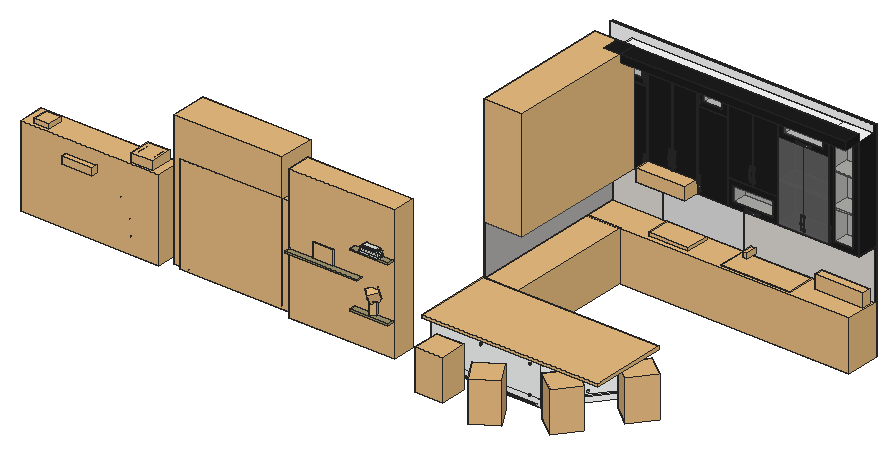
# SketchUp Ruby script. Lengths in inches.
U = 1.inch
M = Sketchup.active_model
def pt(a) = Geom::Point3d.new(a.map { |v| v * U })
def face(e, loops, mat)
  f = e.add_face(loops[0].map { |a| pt(a) })
  loops[1..].each { |l| e.add_face(l.map { |a| pt(a) }).erase! }
  f.material = f.back_material = mat if mat
  f
end
# faces: each face lists its corners as indices into pts; further lists are holes
def faces(e, pts, list, mat = nil) = list.each { |f| face(e, (f[0].is_a?(Array) ? f : [f]).map { |l| l.map { |i| pts[i] } }, mat) }
# xy, xz, yz: faces in a plane at the given z, y or x. An outline is a flat list of corners, or four numbers for a rectangle; further outlines are holes
def ring(l) = l.size == 4 ? [[l[0], l[1]], [l[2], l[1]], [l[2], l[3]], [l[0], l[3]]] : l.each_slice(2).to_a
def flat(e, list, mat, &to3) = list.each { |f| face(e, (f[0].is_a?(Array) ? f : [f]).map { |l| ring(l).map { |u, v| to3.(u, v) } }, mat) }
def xy(e, z, list, mat = nil) = flat(e, list, mat) { |x, y| [x, y, z] }
def xz(e, y, list, mat = nil) = flat(e, list, mat) { |x, z| [x, y, z] }
def yz(e, x, list, mat = nil) = flat(e, list, mat) { |y, z| [x, y, z] }
def lines(e, pts, list) = list.each { |a, b| e.add_line(pt(pts[a]), pt(pts[b])) }
# prism: a flat outline (further loops are holes) pulled along v
def prism(e, loops, v, mat = nil)
  f = face(e, loops, mat); d = Geom::Vector3d.new(v.map { |x| x * U })
  f.pushpull(f.normal.samedirection?(d) ? d.length : -d.length)
end
def box(e, o, s, mat = nil) = prism(e, [[o, [o[0] + s[0], o[1], o[2]], [o[0] + s[0], o[1] + s[1], o[2]], [o[0], o[1] + s[1], o[2]]]], [0, 0, s[2]], mat)
def at(x, y, z, deg = 0) = Geom::Transformation.translation(pt([x, y, z])) * Geom::Transformation.rotation(ORIGIN, Z_AXIS, deg.degrees)
def axes(o, x, y, z) = Geom::Transformation.new([*x, 0, *y, 0, *z, 0, *pt(o).to_a, 1])
def part(name) = M.definitions.add(name)
# library, detail: a bought-in or finely detailed component or shape, given as its bounding box
def library(name, o, s) = part(name).tap { |d| box(d.entities, o, s) }
def detail(e, o, s) = box(e.add_group.entities, o, s)
def put(e, d, t, mat = nil) = e.add_instance(d, t).tap { |i| i.material = mat if mat }
def group(e, t, mat = nil) = e.add_group.tap { |g| g.transformation = t; g.material = mat if mat }.entities
root = M.entities
M.materials.add("Material1 glass").color = [170, 237, 177]
M.materials["Material1 glass"].alpha = 0.04
M.materials.add("Material1 metal").color = [192, 192, 192]
M.materials.add("Material14 kitchen ceramic").color = [29, 29, 29]
M.materials.add("Material17 ceramic").color = [227, 223, 218]
M.materials.add("Material3 mirror").color = [229, 229, 229]
M.materials.add("Material__1").color = [51, 42, 44]
M.materials.add("Material__2").color = [97, 132, 37]
M.materials.add("[ Metal Corrugated Shiny]1").color = [192, 192, 192]
M.materials.add("[Color_000]").color = [255, 255, 255]
M.materials.add("[Color_D05]").color = [255, 242, 204]
M.materials.add("[Translucent Glass Gray]").color = [128, 128, 128]
M.materials["[Translucent Glass Gray]"].alpha = 0.44
M.materials.add("[Wood Lumber ButtJoined]").color = [164, 152, 112]
M.materials.add("[Wood OSB]").color = [240, 195, 122]
M.materials.add("abu metal").color = [255, 255, 255]
M.materials.add("putih ceramic").color = [255, 255, 255]
c1 = library("1-POIGNEE CLC2",[-3.03,-0.375,0],[6.06,0.75,1.42])
c2 = library("Concrete_Pot_w_Mammilleria_Cactus",[-101.61,-9.94,31.01],[5.9,6.21,9.6])
c3 = library("Untitled",[-1.42,-1.51,0],[11.39,11.39,1.78])
c4 = library("Sphere Light",[-10.3,-10.3,-10.3],[20.6,20.6,20.6])
c5 = library("Plants indoor GHD",[-162.85,0,-1.77],[77.96,22.4,70.79])
c6 = part("Wall cabinet door")
box(c6.entities,[-0.79,0,0],[0.79,17.85,60.24],"Material14 kitchen ceramic")
c7 = part("Component\#352")
box(c7.entities,[0,0,0],[0.79,21.46,61.8125],"Material14 kitchen ceramic")
c8 = part("Wall cabinet door \#1")
box(c8.entities,[-0.79,0,0],[0.79,17.76,72.44],"Material14 kitchen ceramic")
c9 = part("Component\#328")
box(c9.entities,[0,0,0],[11.8125,173.23,5.91],"Material14 kitchen ceramic")
c10 = part("Wall cabinet carcass")
xy(c10.entities,11.38,[[0,0,0,188.98,14.76,188.98,14.76,73.29,0.79,73.29,0.79,37.6,14.76,37.6,14.76,15.75,1.97,15.75,1.97,0],[1.97,0,14.76,15.75],[14.76,0,15.75,14.76]],"Material14 kitchen ceramic")
xy(c10.entities,11.8125,[[0,0,0,188.98,14.76,188.98,14.76,73.29,0.79,73.29,0.79,37.6,14.76,37.6,14.76,15.75,1.97,15.75,1.97,0]],"Material14 kitchen ceramic")
xy(c10.entities,12.68,[[0.98,95.93,14.76,130.25],[0.98,168.31,14.76,188.1875]])
xy(c10.entities,13.54,[[0.98,131.23,14.76,166.94]],"Material14 kitchen ceramic")
xy(c10.entities,19.69,[[0.79,37.6,14.76,73.29]],"Material14 kitchen ceramic")
xy(c10.entities,30.63,[[0.98,95.93,14.76,130.25]])
xy(c10.entities,74.02,[[0.98,131.23,14.76,166.94]],"Material14 kitchen ceramic")
xy(c10.entities,74.88,[[0.98,16.73,14.76,36.61],[0.98,74.28,14.76,94.16],[0.98,132.02,14.76,166.54]],"putih ceramic")
xy(c10.entities,91.26,[[0.98,168.31,14.76,188.1875]])
xy(c10.entities,91.26,[[0.98,16.73,14.76,36.61],[0.98,74.28,14.76,94.16],[0.98,132.02,14.76,166.54]],"putih ceramic")
xy(c10.entities,92.52,[[1.97,15.75,14.76,167.52],[1.97,167.52,14.76,188.98]],"putih ceramic")
xy(c10.entities,98.43,[[0,0,1.97,188.98]],"Material14 kitchen ceramic")
xz(c10.entities,0,[[0,11.38,1.97,11.8125],[1.97,11.38,14.76,11.8125],[14.76,11.38,15.75,11.8125]],"Material14 kitchen ceramic")
xz(c10.entities,0,[[0,11.8125,1.97,98.43]],"putih ceramic")
xz(c10.entities,14.76,[[14.76,11.38,15.75,11.8125]],"abu metal")
xz(c10.entities,15.75,[[1.97,11.38,14.76,11.8125]],"Material14 kitchen ceramic")
xz(c10.entities,15.75,[[1.97,11.8125,14.76,92.52]],"putih ceramic")
xz(c10.entities,16.73,[[0.98,74.88,14.76,91.26]],"putih ceramic")
xz(c10.entities,36.61,[[0.98,74.88,14.76,91.26]],"putih ceramic")
xz(c10.entities,37.6,[[0.79,11.38,14.76,11.8125],[0.79,11.8125,14.76,19.69]],"Material14 kitchen ceramic")
xz(c10.entities,73.29,[[0.79,11.38,14.76,11.8125],[0.79,11.8125,14.76,19.69]],"Material14 kitchen ceramic")
xz(c10.entities,74.28,[[0.98,74.88,14.76,91.26]],"putih ceramic")
xz(c10.entities,94.16,[[0.98,74.88,14.76,91.26]],"putih ceramic")
xz(c10.entities,95.93,[[0.98,12.68,14.76,30.63]])
xz(c10.entities,130.25,[[0.98,12.68,14.76,30.63]])
xz(c10.entities,131.23,[[0.98,13.54,14.76,74.02]],"Material14 kitchen ceramic")
xz(c10.entities,132.02,[[0.98,74.88,14.76,91.26]],"putih ceramic")
xz(c10.entities,166.54,[[0.98,74.88,14.76,91.26]],"putih ceramic")
xz(c10.entities,166.94,[[0.98,13.54,14.76,74.02]],"Material14 kitchen ceramic")
xz(c10.entities,168.31,[[0.98,12.68,14.76,91.26]])
xz(c10.entities,188.1875,[[0.98,12.68,14.76,91.26]])
xz(c10.entities,188.98,[[0,11.38,14.76,11.8125],[0,11.8125,0,98.43,1.97,98.43,1.97,92.52,14.76,92.52,14.76,11.8125]],"Material14 kitchen ceramic")
yz(c10.entities,0,[[0,11.38,188.98,11.8125]],"Material14 kitchen ceramic")
yz(c10.entities,0,[[0,11.8125,188.98,98.43]],"putih ceramic")
yz(c10.entities,0.79,[[37.6,11.38,73.29,11.8125],[37.6,11.8125,73.29,19.69]],"Material14 kitchen ceramic")
yz(c10.entities,0.98,[[95.93,12.68,130.25,30.63],[168.31,12.68,188.1875,91.26]])
yz(c10.entities,0.98,[[131.23,13.54,166.94,74.02]],"Material14 kitchen ceramic")
yz(c10.entities,0.98,[[16.73,74.88,36.61,91.26],[74.28,74.88,94.16,91.26],[132.02,74.88,166.54,91.26]],"putih ceramic")
yz(c10.entities,1.97,[[0,11.38,15.75,11.8125]],"Material14 kitchen ceramic")
yz(c10.entities,1.97,[[0,11.8125,15.75,11.8125,15.75,92.52,188.98,92.52,188.98,98.43,0,98.43]],"putih ceramic")
yz(c10.entities,14.76,[[[95.14,11.8125,131.04,31.5],[95.93,12.68,130.25,30.63]],[[167.52,11.8125,188.98,92.125],[168.31,12.68,188.1875,91.26]]])
yz(c10.entities,14.76,[[166.94,11.38,167.52,11.8125],[131.23,11.8125,166.94,13.54]],"Material14 kitchen ceramic")
yz(c10.entities,14.76,[[14.76,11.38,15.75,11.8125],[15.75,11.38,37.6,11.8125],[73.29,11.38,95.14,11.8125],[95.14,11.38,131.04,11.8125],[131.04,11.38,131.23,11.8125],
  [131.23,11.38,166.94,11.8125],[167.52,11.38,188.98,11.8125]],"abu metal")
yz(c10.entities,14.76,[[[15.75,11.8125,37.6,11.8125,37.6,19.69,73.29,19.69,73.29,11.8125,95.14,11.8125,95.14,31.5,131.04,31.5,131.04,11.8125,131.23,11.8125,131.23,92.125,167.32,92.125,167.32,74.02,166.94,74.02,166.94,11.8125,167.52,11.8125,167.52,92.52,15.75,92.52],[15.94,74.02,37.4,92.125],[73.49,74.02,94.95,92.125]],[[15.94,74.02,37.4,92.125],[16.73,74.88,36.61,91.26]],[[73.49,74.02,94.95,92.125],[74.28,74.88,94.16,91.26]],[[131.23,74.02,167.32,92.125],[132.02,74.88,166.54,91.26]],[167.52,92.125,188.98,92.52]],"putih ceramic")
yz(c10.entities,15.75,[[0,11.38,14.76,11.8125]],"Material14 kitchen ceramic")
c11 = part("Cabinet panel")
box(c11.entities,[-0.79,0,0],[0.4,17.76,62],"[Translucent Glass Gray]")
c12 = library("Bosch-Ventilation-DUH30252UC",[0,-0.03,0],[30,20.53,6.0625])
c13 = part("Framed cabinet door")
xy(c13.entities,5.91,[[-0.79,0,0,21.46]],"Material14 kitchen ceramic")
xy(c13.entities,9.84,[[-0.79,3.9375,-0.39,17.52],[-0.39,3.9375,0,17.52]],"Material14 kitchen ceramic")
xy(c13.entities,82.28,[[-0.79,3.9375,-0.39,17.52],[-0.39,3.9375,0,17.52]],"Material14 kitchen ceramic")
xy(c13.entities,86.22,[[-0.79,0,0,21.46]],"Material14 kitchen ceramic")
xz(c13.entities,0,[[-0.79,5.91,0,86.22]],"Material14 kitchen ceramic")
xz(c13.entities,3.9375,[[-0.79,9.84,-0.39,82.28],[-0.39,9.84,0,82.28]],"Material14 kitchen ceramic")
xz(c13.entities,17.52,[[-0.79,9.84,-0.39,82.28],[-0.39,9.84,0,82.28]],"Material14 kitchen ceramic")
xz(c13.entities,21.46,[[-0.79,5.91,0,86.22]],"Material14 kitchen ceramic")
yz(c13.entities,-0.79,[[[0,5.91,21.46,86.22],[3.9375,9.84,17.52,82.28]]],"Material14 kitchen ceramic")
yz(c13.entities,-0.39,[[3.9375,9.84,17.52,82.28]],"[Translucent Glass Gray]")
yz(c13.entities,0,[[[0,5.91,21.46,86.22],[3.9375,9.84,17.52,82.28]]],"Material14 kitchen ceramic")
c14 = part("Framed cabinet front")
xy(c14.entities,0,[[0,0,0.79,21.46]],"Material14 kitchen ceramic")
xy(c14.entities,3.58,[[0,3.9375,0.39,17.52],[0.39,3.9375,0.79,17.52]],"Material14 kitchen ceramic")
xy(c14.entities,12.88,[[0,3.9375,0.39,17.52],[0.39,3.9375,0.79,17.52]],"Material14 kitchen ceramic")
xy(c14.entities,16.46,[[0,0,0.79,21.46]],"Material14 kitchen ceramic")
xz(c14.entities,0,[[0,0,0.79,16.46]],"Material14 kitchen ceramic")
xz(c14.entities,3.9375,[[0,3.58,0.39,12.88],[0.39,3.58,0.79,12.88]],"Material14 kitchen ceramic")
xz(c14.entities,17.52,[[0,3.58,0.39,12.88],[0.39,3.58,0.79,12.88]],"Material14 kitchen ceramic")
xz(c14.entities,21.46,[[0,0,0.79,16.46]],"Material14 kitchen ceramic")
yz(c14.entities,0,[[[0,0,21.46,16.46],[3.9375,3.58,17.52,12.88]]],"Material14 kitchen ceramic")
yz(c14.entities,0.39,[[3.9375,3.58,17.52,12.88]],"[Translucent Glass Gray]")
yz(c14.entities,0.79,[[[0,0,21.46,16.46],[3.9375,3.58,17.52,12.88]]],"Material14 kitchen ceramic")
c15 = part("Framed cabinet front \#1")
xy(c15.entities,0,[[0,0,0.79,21.46]],"Material14 kitchen ceramic")
xy(c15.entities,3.58,[[0,3.9375,0.39,17.52],[0.39,3.9375,0.79,17.52]],"Material14 kitchen ceramic")
xy(c15.entities,12.88,[[0,3.9375,0.39,17.52],[0.39,3.9375,0.79,17.52]],"Material14 kitchen ceramic")
xy(c15.entities,16.46,[[0,0,0.79,21.46]],"Material14 kitchen ceramic")
xz(c15.entities,0,[[0,0,0.79,16.46]],"Material14 kitchen ceramic")
xz(c15.entities,3.9375,[[0,3.58,0.39,12.88],[0.39,3.58,0.79,12.88]],"Material14 kitchen ceramic")
xz(c15.entities,17.52,[[0,3.58,0.39,12.88],[0.39,3.58,0.79,12.88]],"Material14 kitchen ceramic")
xz(c15.entities,21.46,[[0,0,0.79,16.46]],"Material14 kitchen ceramic")
yz(c15.entities,0,[[[0,0,21.46,16.46],[3.9375,3.58,17.52,12.88]]],"Material14 kitchen ceramic")
yz(c15.entities,0.39,[[3.9375,3.58,17.52,12.88]],"[Translucent Glass Gray]")
yz(c15.entities,0.79,[[[0,0,21.46,16.46],[3.9375,3.58,17.52,12.88]]],"Material14 kitchen ceramic")
c16 = part("Framed cabinet front \#2")
xy(c16.entities,0,[[0,0,0.79,35.89]],"Material14 kitchen ceramic")
xy(c16.entities,3.58,[[0,3.9375,0.39,31.96],[0.39,3.9375,0.79,31.96]],"Material14 kitchen ceramic")
xy(c16.entities,14.32,[[0,3.9375,0.39,31.96],[0.39,3.9375,0.79,31.96]],"Material14 kitchen ceramic")
xy(c16.entities,17.9,[[0,0,0.79,35.89]],"Material14 kitchen ceramic")
xz(c16.entities,0,[[0,0,0.79,17.9]],"Material14 kitchen ceramic")
xz(c16.entities,3.9375,[[0,3.58,0.39,14.32],[0.39,3.58,0.79,14.32]],"Material14 kitchen ceramic")
xz(c16.entities,31.96,[[0,3.58,0.39,14.32],[0.39,3.58,0.79,14.32]],"Material14 kitchen ceramic")
xz(c16.entities,35.89,[[0,0,0.79,17.9]],"Material14 kitchen ceramic")
yz(c16.entities,0,[[[0,0,35.89,17.9],[3.9375,3.58,31.96,14.32]]],"Material14 kitchen ceramic")
yz(c16.entities,0.39,[[3.9375,3.58,31.96,14.32]],"[Translucent Glass Gray]")
yz(c16.entities,0.79,[[[0,0,35.89,17.9],[3.9375,3.58,31.96,14.32]]],"Material14 kitchen ceramic")
c17 = part("Framed cabinet front \#3")
xy(c17.entities,0,[[0,0,0.79,36.09]],"Material14 kitchen ceramic")
xy(c17.entities,3.58,[[0,3.9375,0.39,32.15],[0.39,3.9375,0.79,32.15]],"Material14 kitchen ceramic")
xy(c17.entities,12.88,[[0,3.9375,0.39,32.15],[0.39,3.9375,0.79,32.15]],"Material14 kitchen ceramic")
xy(c17.entities,16.46,[[0,0,0.79,36.09]],"Material14 kitchen ceramic")
xz(c17.entities,0,[[0,0,0.79,16.46]],"Material14 kitchen ceramic")
xz(c17.entities,3.9375,[[0,3.58,0.39,12.88],[0.39,3.58,0.79,12.88]],"Material14 kitchen ceramic")
xz(c17.entities,32.15,[[0,3.58,0.39,12.88],[0.39,3.58,0.79,12.88]],"Material14 kitchen ceramic")
xz(c17.entities,36.09,[[0,0,0.79,16.46]],"Material14 kitchen ceramic")
yz(c17.entities,0,[[[0,0,36.09,16.46],[3.9375,3.58,32.15,12.88]]],"Material14 kitchen ceramic")
yz(c17.entities,0.39,[[3.9375,3.58,32.15,12.88]],"[Translucent Glass Gray]")
yz(c17.entities,0.79,[[[0,0,36.09,16.46],[3.9375,3.58,32.15,12.88]]],"Material14 kitchen ceramic")
c18 = part("Group\#24")
xy(c18.entities,0,[[0,0,35.43,15.75],[0,390.79,35.43,406.54]],"[ Metal Corrugated Shiny]1")
xy(c18.entities,7.09,[[0,0,35.43,15.75],[0,390.79,35.43,406.54]],"[ Metal Corrugated Shiny]1")
xz(c18.entities,0,[[0,0,35.43,7.09]],"[ Metal Corrugated Shiny]1")
xz(c18.entities,406.54,[[0,0,35.43,7.09]],"[ Metal Corrugated Shiny]1")
yz(c18.entities,0,[[0,0,0,7.09,15.75,7.09,21.89,7.25,21.89,0.16,15.75,0],[390.79,0,384.65,0.16,384.65,7.25,390.79,7.09,406.54,7.09,406.54,0],[21.89,0.16,21.89,7.25,28.01,7.7,28.01,0.62],[384.65,0.16,378.53,0.62,378.53,7.7,384.65,7.25],[28.01,0.62,28.01,7.7,34.11,8.45,34.11,1.36],
  [378.53,0.62,372.43,1.36,372.43,8.45,378.53,7.7],[34.11,1.36,34.11,8.45,40.16,9.49,40.16,2.4],[372.43,1.36,366.38,2.4,366.38,9.49,372.43,8.45],[40.16,2.4,40.16,9.49,46.15,10.82,46.15,3.73],[366.38,2.4,360.38,3.73,360.38,10.82,366.38,9.49],
  [46.15,3.73,46.15,10.82,52.08,12.43,52.08,5.34],[360.38,3.73,354.46,5.34,354.46,12.43,360.38,10.82],[52.08,5.34,52.08,12.43,57.92,14.32,57.92,7.24],[354.46,5.34,348.62,7.24,348.62,14.32,354.46,12.43],[57.92,7.24,57.92,14.32,63.66,16.5,63.66,9.41],
  [348.62,7.24,342.875,9.41,342.875,16.5,348.62,14.32],[63.66,9.41,63.66,16.5,69.29,18.94,69.29,11.85],[342.875,9.41,337.24,11.85,337.24,18.94,342.875,16.5],[69.29,11.85,69.29,18.94,74.8,21.65,74.8,14.57],[337.24,11.85,331.73,14.57,331.73,21.65,337.24,18.94],
  [74.8,14.57,74.8,21.65,99.35,31.6,99.35,24.52],[331.73,14.57,307.1875,24.52,307.1875,31.6,331.73,21.65],[99.35,24.52,99.35,31.6,124.66,39.42,124.66,32.33],[307.1875,24.52,281.88,32.33,281.88,39.42,307.1875,31.6],[124.66,32.33,124.66,39.42,150.54,45.04,150.54,37.96],
  [281.88,32.33,256,37.96,256,45.04,281.88,39.42],[150.54,37.96,150.54,45.04,176.81,48.43,176.81,41.35],[256,37.96,229.73,41.35,229.73,48.43,256,45.04],[176.81,41.35,176.81,48.43,203.27,49.57,203.27,42.48],[229.73,41.35,203.27,42.48,203.27,49.57,229.73,48.43]],"[ Metal Corrugated Shiny]1")
yz(c18.entities,35.43,[[0,0,15.75,0,21.89,0.16,21.89,7.25,15.75,7.09,0,7.09],[390.79,0,406.54,0,406.54,7.09,390.79,7.09,384.65,7.25,384.65,0.16],[21.89,0.16,28.01,0.62,28.01,7.7,21.89,7.25],[384.65,0.16,384.65,7.25,378.53,7.7,378.53,0.62],[28.01,0.62,34.11,1.36,34.11,8.45,28.01,7.7],
  [378.53,0.62,378.53,7.7,372.43,8.45,372.43,1.36],[34.11,1.36,40.16,2.4,40.16,9.49,34.11,8.45],[372.43,1.36,372.43,8.45,366.38,9.49,366.38,2.4],[40.16,2.4,46.15,3.73,46.15,10.82,40.16,9.49],[366.38,2.4,366.38,9.49,360.38,10.82,360.38,3.73],
  [46.15,3.73,52.08,5.34,52.08,12.43,46.15,10.82],[360.38,3.73,360.38,10.82,354.46,12.43,354.46,5.34],[52.08,5.34,57.92,7.24,57.92,14.32,52.08,12.43],[354.46,5.34,354.46,12.43,348.62,14.32,348.62,7.24],[57.92,7.24,63.66,9.41,63.66,16.5,57.92,14.32],
  [348.62,7.24,348.62,14.32,342.875,16.5,342.875,9.41],[63.66,9.41,69.29,11.85,69.29,18.94,63.66,16.5],[342.875,9.41,342.875,16.5,337.24,18.94,337.24,11.85],[69.29,11.85,74.8,14.57,74.8,21.65,69.29,18.94],[337.24,11.85,337.24,18.94,331.73,21.65,331.73,14.57],
  [74.8,14.57,99.35,24.52,99.35,31.6,74.8,21.65],[331.73,14.57,331.73,21.65,307.1875,31.6,307.1875,24.52],[99.35,24.52,124.66,32.33,124.66,39.42,99.35,31.6],[307.1875,24.52,307.1875,31.6,281.88,39.42,281.88,32.33],[124.66,32.33,150.54,37.96,150.54,45.04,124.66,39.42],
  [281.88,32.33,281.88,39.42,256,45.04,256,37.96],[150.54,37.96,176.81,41.35,176.81,48.43,150.54,45.04],[256,37.96,256,45.04,229.73,48.43,229.73,41.35],[176.81,41.35,203.27,42.48,203.27,49.57,176.81,48.43],[229.73,41.35,229.73,48.43,203.27,49.57,203.27,42.48]],"[ Metal Corrugated Shiny]1")
p = [[35.43,15.75,0],[0,15.75,0],[0,21.89,0.16],[35.43,21.89,0.16],[35.43,384.65,0.16],[0,384.65,0.16],
  [0,390.79,0],[35.43,390.79,0],[0,28.01,0.62],[35.43,28.01,0.62],[35.43,378.53,0.62],[0,378.53,0.62],
  [0,34.11,1.36],[35.43,34.11,1.36],[35.43,372.43,1.36],[0,372.43,1.36],[0,40.16,2.4],[35.43,40.16,2.4],
  [35.43,366.38,2.4],[0,366.38,2.4],[0,46.15,3.73],[35.43,46.15,3.73],[35.43,360.38,3.73],[0,360.38,3.73],
  [0,52.08,5.34],[35.43,52.08,5.34],[35.43,354.46,5.34],[0,354.46,5.34],[0,57.92,7.24],[35.43,57.92,7.24],
  [35.43,348.62,7.24],[0,348.62,7.24],[0,15.75,7.09],[35.43,15.75,7.09],[35.43,21.89,7.25],[0,21.89,7.25],
  [0,384.65,7.25],[35.43,384.65,7.25],[35.43,390.79,7.09],[0,390.79,7.09],[35.43,28.01,7.7],[0,28.01,7.7],
  [0,63.66,9.41],[35.43,63.66,9.41],[35.43,342.875,9.41],[0,342.875,9.41],[0,378.53,7.7],[35.43,378.53,7.7],
  [35.43,34.11,8.45],[0,34.11,8.45],[0,372.43,8.45],[35.43,372.43,8.45],[35.43,40.16,9.49],[0,40.16,9.49],
  [0,366.38,9.49],[35.43,366.38,9.49],[0,69.29,11.85],[35.43,69.29,11.85],[35.43,337.24,11.85],[0,337.24,11.85],
  [35.43,46.15,10.82],[0,46.15,10.82],[0,360.38,10.82],[35.43,360.38,10.82],[35.43,52.08,12.43],[0,52.08,12.43],
  [0,354.46,12.43],[35.43,354.46,12.43],[0,74.8,14.57],[35.43,74.8,14.57],[35.43,331.73,14.57],[0,331.73,14.57],
  [35.43,57.92,14.32],[0,57.92,14.32],[0,348.62,14.32],[35.43,348.62,14.32],[35.43,63.66,16.5],[0,63.66,16.5],
  [0,342.875,16.5],[35.43,342.875,16.5],[0,99.35,24.52],[35.43,99.35,24.52],[35.43,307.1875,24.52],[0,307.1875,24.52],
  [35.43,69.29,18.94],[0,69.29,18.94],[0,337.24,18.94],[35.43,337.24,18.94],[35.43,74.8,21.65],[0,74.8,21.65],
  [0,331.73,21.65],[35.43,331.73,21.65],[35.43,99.35,31.6],[0,99.35,31.6],[0,307.1875,31.6],[35.43,307.1875,31.6],
  [0,124.66,32.33],[35.43,124.66,32.33],[35.43,281.88,32.33],[0,281.88,32.33],[35.43,124.66,39.42],[0,124.66,39.42],
  [0,281.88,39.42],[35.43,281.88,39.42],[0,150.54,37.96],[35.43,150.54,37.96],[35.43,256,37.96],[0,256,37.96],
  [0,176.81,41.35],[35.43,176.81,41.35],[35.43,229.73,41.35],[0,229.73,41.35],[35.43,150.54,45.04],[0,150.54,45.04],
  [0,256,45.04],[35.43,256,45.04],[0,203.27,42.48],[35.43,203.27,42.48],[35.43,176.81,48.43],[0,176.81,48.43],
  [0,229.73,48.43],[35.43,229.73,48.43],[35.43,203.27,49.57],[0,203.27,49.57]]
faces(c18.entities,p,[[0,1,2,3],[4,5,6,7],[3,2,8,9],[10,11,5,4],[9,8,12,13],[14,15,11,10],[13,12,16,17],[18,19,15,14],
  [17,16,20,21],[22,23,19,18],[21,20,24,25],[26,27,23,22],[25,24,28,29],[30,31,27,26],[32,33,34,35],[36,37,38,39],
  [35,34,40,41],[29,28,42,43],[44,45,31,30],[46,47,37,36],[41,40,48,49],[50,51,47,46],[49,48,52,53],[54,55,51,50],
  [43,42,56,57],[58,59,45,44],[53,52,60,61],[62,63,55,54],[61,60,64,65],[66,67,63,62],[57,56,68,69],[70,71,59,58],
  [65,64,72,73],[74,75,67,66],[73,72,76,77],[78,79,75,74],[69,68,80,81],[82,83,71,70],[77,76,84,85],[86,87,79,78],
  [85,84,88,89],[90,91,87,86],[89,88,92,93],[94,95,91,90],[81,80,96,97],[98,99,83,82],[93,92,100,101],[102,103,95,94],
  [97,96,104,105],[106,107,99,98],[105,104,108,109],[110,111,107,106],[101,100,112,113],[114,115,103,102],[109,108,116,117],[117,116,111,110],
  [113,112,118,119],[120,121,115,114],[119,118,122,123],[123,122,121,120]],"[ Metal Corrugated Shiny]1")
c19 = part("Group\#22")
xy(c19.entities,0,[[0,0,35.43,15.75],[0,390.79,35.43,406.54]],"[ Metal Corrugated Shiny]1")
xy(c19.entities,7.09,[[0,0,35.43,15.75],[0,390.79,35.43,406.54]],"[ Metal Corrugated Shiny]1")
xz(c19.entities,0,[[0,0,35.43,7.09]],"[ Metal Corrugated Shiny]1")
xz(c19.entities,406.54,[[0,0,35.43,7.09]],"[ Metal Corrugated Shiny]1")
yz(c19.entities,0,[[0,0,0,7.09,15.75,7.09,21.89,7.25,21.89,0.16,15.75,0],[390.79,0,384.65,0.16,384.65,7.25,390.79,7.09,406.54,7.09,406.54,0],[21.89,0.16,21.89,7.25,28.01,7.7,28.01,0.62],[384.65,0.16,378.53,0.62,378.53,7.7,384.65,7.25],[28.01,0.62,28.01,7.7,34.11,8.45,34.11,1.36],
  [378.53,0.62,372.43,1.36,372.43,8.45,378.53,7.7],[34.11,1.36,34.11,8.45,40.16,9.49,40.16,2.4],[372.43,1.36,366.38,2.4,366.38,9.49,372.43,8.45],[40.16,2.4,40.16,9.49,46.15,10.82,46.15,3.73],[366.38,2.4,360.38,3.73,360.38,10.82,366.38,9.49],
  [46.15,3.73,46.15,10.82,52.08,12.43,52.08,5.34],[360.38,3.73,354.46,5.34,354.46,12.43,360.38,10.82],[52.08,5.34,52.08,12.43,57.92,14.32,57.92,7.24],[354.46,5.34,348.62,7.24,348.62,14.32,354.46,12.43],[57.92,7.24,57.92,14.32,63.66,16.5,63.66,9.41],
  [348.62,7.24,342.875,9.41,342.875,16.5,348.62,14.32],[63.66,9.41,63.66,16.5,69.29,18.94,69.29,11.85],[342.875,9.41,337.24,11.85,337.24,18.94,342.875,16.5],[69.29,11.85,69.29,18.94,74.8,21.65,74.8,14.57],[337.24,11.85,331.73,14.57,331.73,21.65,337.24,18.94],
  [74.8,14.57,74.8,21.65,99.35,31.6,99.35,24.52],[331.73,14.57,307.1875,24.52,307.1875,31.6,331.73,21.65],[99.35,24.52,99.35,31.6,124.66,39.42,124.66,32.33],[307.1875,24.52,281.88,32.33,281.88,39.42,307.1875,31.6],[124.66,32.33,124.66,39.42,150.54,45.04,150.54,37.96],
  [281.88,32.33,256,37.96,256,45.04,281.88,39.42],[150.54,37.96,150.54,45.04,176.81,48.43,176.81,41.35],[256,37.96,229.73,41.35,229.73,48.43,256,45.04],[176.81,41.35,176.81,48.43,203.27,49.57,203.27,42.48],[229.73,41.35,203.27,42.48,203.27,49.57,229.73,48.43]],"[ Metal Corrugated Shiny]1")
yz(c19.entities,35.43,[[0,0,15.75,0,21.89,0.16,21.89,7.25,15.75,7.09,0,7.09],[390.79,0,406.54,0,406.54,7.09,390.79,7.09,384.65,7.25,384.65,0.16],[21.89,0.16,28.01,0.62,28.01,7.7,21.89,7.25],[384.65,0.16,384.65,7.25,378.53,7.7,378.53,0.62],[28.01,0.62,34.11,1.36,34.11,8.45,28.01,7.7],
  [378.53,0.62,378.53,7.7,372.43,8.45,372.43,1.36],[34.11,1.36,40.16,2.4,40.16,9.49,34.11,8.45],[372.43,1.36,372.43,8.45,366.38,9.49,366.38,2.4],[40.16,2.4,46.15,3.73,46.15,10.82,40.16,9.49],[366.38,2.4,366.38,9.49,360.38,10.82,360.38,3.73],
  [46.15,3.73,52.08,5.34,52.08,12.43,46.15,10.82],[360.38,3.73,360.38,10.82,354.46,12.43,354.46,5.34],[52.08,5.34,57.92,7.24,57.92,14.32,52.08,12.43],[354.46,5.34,354.46,12.43,348.62,14.32,348.62,7.24],[57.92,7.24,63.66,9.41,63.66,16.5,57.92,14.32],
  [348.62,7.24,348.62,14.32,342.875,16.5,342.875,9.41],[63.66,9.41,69.29,11.85,69.29,18.94,63.66,16.5],[342.875,9.41,342.875,16.5,337.24,18.94,337.24,11.85],[69.29,11.85,74.8,14.57,74.8,21.65,69.29,18.94],[337.24,11.85,337.24,18.94,331.73,21.65,331.73,14.57],
  [74.8,14.57,99.35,24.52,99.35,31.6,74.8,21.65],[331.73,14.57,331.73,21.65,307.1875,31.6,307.1875,24.52],[99.35,24.52,124.66,32.33,124.66,39.42,99.35,31.6],[307.1875,24.52,307.1875,31.6,281.88,39.42,281.88,32.33],[124.66,32.33,150.54,37.96,150.54,45.04,124.66,39.42],
  [281.88,32.33,281.88,39.42,256,45.04,256,37.96],[150.54,37.96,176.81,41.35,176.81,48.43,150.54,45.04],[256,37.96,256,45.04,229.73,48.43,229.73,41.35],[176.81,41.35,203.27,42.48,203.27,49.57,176.81,48.43],[229.73,41.35,229.73,48.43,203.27,49.57,203.27,42.48]],"[ Metal Corrugated Shiny]1")
p = [[35.43,15.75,0],[0,15.75,0],[0,21.89,0.16],[35.43,21.89,0.16],[35.43,384.65,0.16],[0,384.65,0.16],
  [0,390.79,0],[35.43,390.79,0],[0,28.01,0.62],[35.43,28.01,0.62],[35.43,378.53,0.62],[0,378.53,0.62],
  [0,34.11,1.36],[35.43,34.11,1.36],[35.43,372.43,1.36],[0,372.43,1.36],[0,40.16,2.4],[35.43,40.16,2.4],
  [35.43,366.38,2.4],[0,366.38,2.4],[0,46.15,3.73],[35.43,46.15,3.73],[35.43,360.38,3.73],[0,360.38,3.73],
  [0,52.08,5.34],[35.43,52.08,5.34],[35.43,354.46,5.34],[0,354.46,5.34],[0,57.92,7.24],[35.43,57.92,7.24],
  [35.43,348.62,7.24],[0,348.62,7.24],[0,15.75,7.09],[35.43,15.75,7.09],[35.43,21.89,7.25],[0,21.89,7.25],
  [0,384.65,7.25],[35.43,384.65,7.25],[35.43,390.79,7.09],[0,390.79,7.09],[35.43,28.01,7.7],[0,28.01,7.7],
  [0,63.66,9.41],[35.43,63.66,9.41],[35.43,342.875,9.41],[0,342.875,9.41],[0,378.53,7.7],[35.43,378.53,7.7],
  [35.43,34.11,8.45],[0,34.11,8.45],[0,372.43,8.45],[35.43,372.43,8.45],[35.43,40.16,9.49],[0,40.16,9.49],
  [0,366.38,9.49],[35.43,366.38,9.49],[0,69.29,11.85],[35.43,69.29,11.85],[35.43,337.24,11.85],[0,337.24,11.85],
  [35.43,46.15,10.82],[0,46.15,10.82],[0,360.38,10.82],[35.43,360.38,10.82],[35.43,52.08,12.43],[0,52.08,12.43],
  [0,354.46,12.43],[35.43,354.46,12.43],[0,74.8,14.57],[35.43,74.8,14.57],[35.43,331.73,14.57],[0,331.73,14.57],
  [35.43,57.92,14.32],[0,57.92,14.32],[0,348.62,14.32],[35.43,348.62,14.32],[35.43,63.66,16.5],[0,63.66,16.5],
  [0,342.875,16.5],[35.43,342.875,16.5],[0,99.35,24.52],[35.43,99.35,24.52],[35.43,307.1875,24.52],[0,307.1875,24.52],
  [35.43,69.29,18.94],[0,69.29,18.94],[0,337.24,18.94],[35.43,337.24,18.94],[35.43,74.8,21.65],[0,74.8,21.65],
  [0,331.73,21.65],[35.43,331.73,21.65],[35.43,99.35,31.6],[0,99.35,31.6],[0,307.1875,31.6],[35.43,307.1875,31.6],
  [0,124.66,32.33],[35.43,124.66,32.33],[35.43,281.88,32.33],[0,281.88,32.33],[35.43,124.66,39.42],[0,124.66,39.42],
  [0,281.88,39.42],[35.43,281.88,39.42],[0,150.54,37.96],[35.43,150.54,37.96],[35.43,256,37.96],[0,256,37.96],
  [0,176.81,41.35],[35.43,176.81,41.35],[35.43,229.73,41.35],[0,229.73,41.35],[35.43,150.54,45.04],[0,150.54,45.04],
  [0,256,45.04],[35.43,256,45.04],[0,203.27,42.48],[35.43,203.27,42.48],[35.43,176.81,48.43],[0,176.81,48.43],
  [0,229.73,48.43],[35.43,229.73,48.43],[35.43,203.27,49.57],[0,203.27,49.57]]
faces(c19.entities,p,[[0,1,2,3],[4,5,6,7],[3,2,8,9],[10,11,5,4],[9,8,12,13],[14,15,11,10],[13,12,16,17],[18,19,15,14],
  [17,16,20,21],[22,23,19,18],[21,20,24,25],[26,27,23,22],[25,24,28,29],[30,31,27,26],[32,33,34,35],[36,37,38,39],
  [35,34,40,41],[29,28,42,43],[44,45,31,30],[46,47,37,36],[41,40,48,49],[50,51,47,46],[49,48,52,53],[54,55,51,50],
  [43,42,56,57],[58,59,45,44],[53,52,60,61],[62,63,55,54],[61,60,64,65],[66,67,63,62],[57,56,68,69],[70,71,59,58],
  [65,64,72,73],[74,75,67,66],[73,72,76,77],[78,79,75,74],[69,68,80,81],[82,83,71,70],[77,76,84,85],[86,87,79,78],
  [85,84,88,89],[90,91,87,86],[89,88,92,93],[94,95,91,90],[81,80,96,97],[98,99,83,82],[93,92,100,101],[102,103,95,94],
  [97,96,104,105],[106,107,99,98],[105,104,108,109],[110,111,107,106],[101,100,112,113],[114,115,103,102],[109,108,116,117],[117,116,111,110],
  [113,112,118,119],[120,121,115,114],[119,118,122,123],[123,122,121,120]],"[ Metal Corrugated Shiny]1")
c20 = part("Wall cabinet run")
box(c20.entities,[14.96,73.49,0],[0.79,21.46,61.8125],"Material14 kitchen ceramic")
put(c20.entities,c6,at(15.75,95.14,20.08))
put(c20.entities,c6,at(15.75,113.2,20.08))
put(c20.entities,c7,at(14.96,15.94,0))
put(c20.entities,c8,at(15.75,55.55,7.875))
put(c20.entities,c8,at(15.75,37.6,7.875))
put(c20.entities,c9,at(15.75,15.75,80.71))
put(c20.entities,c10,at(0,0,-11.8125))
put(c20.entities,c11,at(15.75,131.23,0))
put(c20.entities,c11,at(15.75,149.1875,0))
put(c20.entities,c12,axes([26.36,38.19,0],[0,1.17,0],[-1.17,0,0],[0,0,1.5795]))
put(c20.entities,c13,at(15.75,167.52,-5.91))
put(c20.entities,c14,axes([14.96,73.49,62.2],[1,0,0],[0,1,0],[0,0,1.1]))
put(c20.entities,c15,axes([14.96,15.94,62.2],[1,0,0],[0,1,0],[0,0,1.1]))
put(c20.entities,c16,axes([14.96,95.14,0],[1,0,0],[0,1,0],[0,0,1.1]))
put(c20.entities,c17,axes([14.96,131.23,62.2],[1,0,0],[0,1,0],[0,0,1.1]))
put(c20.entities,c18,axes([15.75,168.11,2.03],[0,0.02199,0],[0,0,0.02878],[0.02199,0,0]))
put(c20.entities,c18,axes([15.35,149.8,2.03],[0,0.02199,0],[0,0,0.02878],[0.02199,0,0]))
put(c20.entities,c19,axes([15.35,147.64,2.03],[0,0.02199,0],[0,0,0.02878],[0.02199,0,0]))
put(c20.entities,c19,axes([15.75,74.8,2.03],[0,0.02199,0],[0,0,0.02878],[0.02199,0,0]))
put(c20.entities,c19,axes([15.75,35.39,2.03],[0,0.02199,0],[0,0,0.02878],[0.02199,0,0]))
put(c20.entities,c19,axes([15.75,111.15,22.77],[0,0.02199,0],[0,0,0.02878],[0.02199,0,0]))
put(c20.entities,c19,axes([15.75,113.86,22.77],[0,0.02199,0],[0,0,0.02878],[0.02199,0,0]))
put(c20.entities,c19,axes([15.75,56.9,12.12],[0,0.02199,0],[0,0,0.02878],[0.02199,0,0]))
put(c20.entities,c19,axes([15.75,53.43,12.12],[0,0.02199,0],[0,0,0.02878],[0.02199,0,0]))
put(c20.entities,c19,axes([15.75,107.58,2.36],[0,0,-0.02419],[0,0.02617,0],[0.02199,0,0]))
put(c20.entities,c19,axes([15.75,143.92,64.63],[0,0,-0.02419],[0,0.02617,0],[0.02199,0,0]))
put(c20.entities,c19,axes([15.75,35.39,64.01],[0,0.02199,0],[0,0,0.02878],[0.02199,0,0]))
put(c20.entities,c19,axes([15.75,74.65,64.01],[0,0.02199,0],[0,0,0.02878],[0.02199,0,0]))
c21 = library("Wall cabinet run \#1",[0,0,-0.43],[99.61,27.56,87.04])
c22 = library("Base cabinet run \#1",[0,0,0],[91.73,24.71,35.43])
c23 = library("Base cabinet run",[0,0,0],[24.71,188.98,35.43])
c24 = part("Component\#350")
xy(c24.entities,0,[[0,0,1.57,1.57],[0,1.57,1.57,188.98]],"putih ceramic")
xy(c24.entities,35.43,[[0,0,1.57,1.57],[0,1.57,1.57,188.98]],"putih ceramic")
xz(c24.entities,0,[[0,0,1.57,35.43]],"putih ceramic")
xz(c24.entities,1.57,[[0,0,1.57,35.43]],"putih ceramic")
xz(c24.entities,188.98,[[0,0,1.57,35.43]],"Material14 kitchen ceramic")
yz(c24.entities,0,[[0,0,1.57,35.43],[1.57,0,188.98,35.43]],"putih ceramic")
yz(c24.entities,1.57,[[0,0,1.57,35.43]],"Material14 kitchen ceramic")
yz(c24.entities,1.57,[[1.57,0,188.98,35.43]],"Material17 ceramic")
c25 = part("Component\#387")
xy(c25.entities,0,[[0,0,113.78,1.57]],"Material14 kitchen ceramic")
xy(c25.entities,35.43,[[0,0,113.78,1.57]],"Material14 kitchen ceramic")
xz(c25.entities,0,[[0,0,113.78,35.43]],"Material14 kitchen ceramic")
xz(c25.entities,1.57,[[0,0,113.78,35.43]],"Material17 ceramic")
yz(c25.entities,0,[[0,0,1.57,35.43]],"Material14 kitchen ceramic")
yz(c25.entities,113.78,[[0,0,1.57,35.43]],"Material14 kitchen ceramic")
c26 = part("Component\#33")
prism(c26.entities,[[[0.91,0.01,0.74],[0.87,0.05,0.89],[0.79,0.11,1.01],[0.7,0.18,1.1],[0.58,0.27,1.16],[0.46,0.36,1.18],[0.34,0.46,1.16],[0.23,0.55,1.1],[0.14,0.62,1.01],[0.0625,0.68,0.89],[0.02,0.72,0.74],[0,0.73,0.59],[0.02,0.72,0.4375],[0.0625,0.68,0.3],[0.14,0.62,0.17],[0.23,0.55,0.08],[0.34,0.46,0.02],[0.46,0.36,0],[0.58,0.27,0.02],[0.7,0.18,0.08],[0.79,0.11,0.17],[0.87,0.05,0.3],[0.91,0.01,0.4375],[0.93,0,0.59]]],[0.12,0.15,0],"Material1 metal")
c27 = library("coz_ll_125-50",[0,0,0],[49.21,19.69,5.91])
c28 = part("Component\#436")
prism(c28.entities,[[[0,1.96,0.29],[0,1.71,0.12],[0,1.41,0.02],[0,1.11,0],[0,0.8,0.06],[0,0.53,0.19],[0,0.29,0.4],[0,0.12,0.65],[0,0.02,0.94],[0,0,1.25],[0,0.06,1.55],[0,0.19,1.83],[0,0.4,2.0625],[0,0.65,2.24],[0,0.94,2.34],[0,1.25,2.36],[0,1.55,2.3],[0,1.83,2.16],[0,2.0625,1.96],[0,2.24,1.71],[0,2.34,1.41],[0,2.36,1.11],[0,2.3,0.8],[0,2.16,0.53]]],[0.12,0,0],"abu metal")
c29 = library("Deca_Torneira+Lavatorio+Clean_1178.C.CLN_Parede",[5.41,0,8.81],[3.41,8.24,3.84])
c30 = part("Component\#432")
box(c30.entities,[-13.78,0,0],[13.78,19.88,0.79])
c31 = part("Component\#435")
box(c31.entities,[0,0,0],[113.78,0.2,35.43],"[Translucent Glass Gray]")
c32 = library("Sem+nome",[12.38,5.35,0],[34.47,6.17,9.61])
c33 = library("Gas cooktop",[0,0,0],[28.35,16.54,1.98])
c34 = part("Component\#433")
box(c34.entities,[0,0,0],[13.78,35.71,0.79],"Material14 kitchen ceramic")
c35 = part("Component\#24")
xy(c35.entities,0,[[0,0,0.39,78.5]],"Material1 glass")
xy(c35.entities,27.95,[[0,0,0.39,78.5]],"Material1 glass")
xz(c35.entities,0,[[0,0,0.39,27.95]],"Material1 glass")
xz(c35.entities,78.5,[[0,0,0.39,27.95]],"Material1 glass")
yz(c35.entities,0.39,[[0,0,78.5,27.95]],"Material1 glass")
c36 = part("Component\#434")
xy(c36.entities,0,[[0,0,0.2,57.55]],"abu metal")
xy(c36.entities,35.43,[[0,0,0.2,57.55]],"abu metal")
xz(c36.entities,0,[[0,0,0.2,35.43]],"abu metal")
xz(c36.entities,57.55,[[0,0,0.2,35.43]],"abu metal")
yz(c36.entities,0,[[0,0,57.55,35.43]],"abu metal")
yz(c36.entities,0.2,[[0,0,57.55,35.43]],"Material3 mirror")
c37 = part("Component\#437")
prism(c37.entities,[[[0.59,0,2.2],[0.35,0,2.02],[0.16,0,1.77],[0.04,0,1.49],[0,0,1.18],[0.04,0,0.875],[0.16,0,0.59],[0.35,0,0.35],[0.59,0,0.16],[0.875,0,0.04],[1.18,0,0],[1.49,0,0.04],[1.77,0,0.16],[2.02,0,0.35],[2.2,0,0.59],[2.32,0,0.875],[2.36,0,1.18],[2.32,0,1.49],[2.2,0,1.77],[2.02,0,2.02],[1.77,0,2.2],[1.49,0,2.32],[1.18,0,2.36],[0.875,0,2.32]]],[0,0.47,0],"abu metal")
c38 = part("Component\#27")
prism(c38.entities,[[[46.85,0,0],[23.23,0,0],[23.23,67.26,0],[0,85.51,0],[0,115.55,0],[46.85,78.74,0]]],[0,0,33.07],"putih ceramic")
c39 = part("Component\#28")
xy(c39.entities,0,[[46.66,-0.1,0,36.57,0.24,36.88,46.91,0.21]],"Material1 glass")
xy(c39.entities,27.95,[[46.66,-0.1,46.91,0.21,0.24,36.88,0,36.57]],"Material1 glass")
p = [[46.91,0.21,0],[46.91,0.21,27.95],[46.66,-0.1,27.95],[46.66,-0.1,0],[0.24,36.88,27.95],[0.24,36.88,0],
  [0,36.57,0],[0,36.57,27.95]]
faces(c39.entities,p,[[0,1,2,3],[4,1,0,5],[4,5,6,7]],"Material1 glass")
c40 = library("Island countertop",[0,0,0],[54.72,125.67,2.36])
c41 = library("HMI+SHE+SAID+BARSTOOL",[-9.1,-9.7,0],[19.23,19.64,34.25])
c42 = part("Component\#31")
prism(c42.entities,[[[0,0.17,1.01],[0,0.3,1.1],[0,0.4375,1.16],[0,0.59,1.18],[0,0.74,1.16],[0,0.89,1.1],[0,1.01,1.01],[0,1.1,0.89],[0,1.16,0.74],[0,1.18,0.59],[0,1.16,0.4375],[0,1.1,0.3],[0,1.01,0.17],[0,0.89,0.08],[0,0.74,0.02],[0,0.59,0],[0,0.4375,0.02],[0,0.3,0.08],[0,0.17,0.17],[0,0.08,0.3],[0,0.02,0.4375],[0,0,0.59],[0,0.02,0.74],[0,0.08,0.89]]],[0.2,0,0],"Material1 metal")
c43 = part("Component\#21")
box(c43.entities,[0,0,0],[0.59,79.03,0.79],"putih ceramic")
c44 = part("Kitchen with island")
xy(c44.entities,3.9375,[[162.82,78.76,115.75,115.75,116.11,116.21,163.1875,79.22]],"putih ceramic")
xy(c44.entities,4.72,[[162.82,78.76,163.1875,79.22,116.11,116.21,115.75,115.75,162.6,78.9375]],"putih ceramic")
p = [[115.75,115.75,4.72],[115.75,115.75,3.9375],[162.82,78.76,3.9375],[162.82,78.76,4.72],[162.6,78.9375,4.72],[167.27,78.75,4.72],
  [167.27,78.75,3.9375],[167.64,79.22,3.9375],[167.64,79.22,4.72],[116.11,116.21,3.9375],[116.11,116.21,4.72],[163.1875,79.22,4.72],
  [163.1875,79.22,3.9375],[167.05,78.93,4.72]]
faces(c44.entities,p,[[0,1,2,3,4],[5,6,7,8],[9,10,11,12],[1,0,10,9]],"putih ceramic")
lines(c44.entities,p,[[13,5]])
put(c44.entities,c20,axes([0,0,70.87],[1,0,0],[0,1,0],[0,0,0.90909]))
put(c44.entities,c21,axes([15.75,0,70.87],[1,0,0],[0,1,0],[0,0,0.90909]))
put(c44.entities,c22,at(23.62,0,0))
put(c44.entities,c23,at(0,0,0))
put(c44.entities,c24,at(0,0,35.43))
put(c44.entities,c25,at(1.57,0,35.43))
put(c44.entities,c26,at(118.78,113.14,8.27))
put(c44.entities,c26,at(118.78,113.14,28.35))
put(c44.entities,c27,at(22.06,95.28,29.74,90))
put(c44.entities,c28,at(1.57,173.66,61.8125))
put(c44.entities,c29,axes([9.37,95.5,28.63],[0,0.9471,0],[-0.9471,0,0],[0,0,0.9471]))
put(c44.entities,c28,at(1.57,18.7,61.8125))
put(c44.entities,c30,at(14.76,168.31,119.01))
put(c44.entities,c31,at(1.57,1.46,35.43))
put(c44.entities,c32,at(-1,200.28,35.43,-90))
put(c44.entities,c30,at(14.76,168.31,94.93))
put(c44.entities,c28,at(1.57,110.28,61.8125))
put(c44.entities,c28,at(1.57,142.13,61.8125))
put(c44.entities,c33,at(20.68,42.52,35.43,90))
put(c44.entities,c34,at(0.98,131.23,99.53))
put(c44.entities,c35,at(162.6,0.39,4.92))
put(c44.entities,c36,at(1.57,37.6,35.43))
put(c44.entities,c37,at(95.8,1.26,61.8125))
put(c44.entities,c38,at(115.75,0.2,0))
put(c44.entities,c37,at(15.32,1.26,61.8125))
put(c44.entities,c39,at(115.9,79.06,4.92))
put(c44.entities,c40,at(115.75,0,33.07))
put(c44.entities,c41,axes([133.96,126.09,0],[-0.61782,-0.78632,0],[0.78632,-0.61782,0],[0,0,0.85]))
put(c44.entities,c37,at(56.03,1.26,61.8125))
put(c44.entities,c42,at(162.99,3.74,28.35))
put(c44.entities,c41,axes([189.62,61.15,0],[-0.53288,0.84619,0],[-0.84619,-0.53288,0],[0,0,0.85]))
put(c44.entities,c26,at(163.57,81.43,28.35))
put(c44.entities,c42,at(167.4375,74.21,8.27))
put(c44.entities,c26,at(143.42,97.27,28.35))
put(c44.entities,c42,at(167.4375,38.97,28.35))
put(c44.entities,c42,at(167.4375,3.74,8.27))
put(c44.entities,c26,at(163.57,81.43,8.27))
put(c44.entities,c42,at(167.4375,38.97,8.27))
put(c44.entities,c26,at(143.42,97.27,8.27))
put(c44.entities,c41,axes([183.65,22.75,0],[-1,0,0],[0,-1,0],[0,0,0.85]))
put(c44.entities,c42,at(167.4375,74.21,28.35))
put(c44.entities,c43,at(167.05,0.19,3.9375))
put(c44.entities,c41,axes([170.29,101.04,0],[-0.61782,-0.78632,0],[0.78632,-0.61782,0],[0,0,0.85]))
c45 = part("Upright book \#1")
xy(c45.entities,0,[[0.12,0.12,1.66,6.72]])
xy(c45.entities,0,[[0,0,0,6.8,0.12,6.8,0.12,0.12,1.66,0.12,1.66,6.8,1.77,6.8,1.77,0]],"[Color_000]")
xy(c45.entities,9.22,[[0.12,0.12,1.66,6.72]],"[Color_D05]")
xy(c45.entities,9.33,[[0,0,1.77,0,1.77,6.8,1.66,6.8,1.66,0.12,0.12,0.12,0.12,6.8,0,6.8]],"[Color_000]")
xz(c45.entities,0,[[0,0,1.77,9.33]])
xz(c45.entities,0.12,[[0.12,0,1.66,9.22]])
xz(c45.entities,0.12,[[0.12,9.22,1.66,9.33]],"[Color_000]")
xz(c45.entities,6.72,[[0.12,0,1.66,9.22]],"[Color_D05]")
xz(c45.entities,6.8,[[0,0,0.12,9.33],[1.66,0,1.77,9.33]],"[Color_000]")
yz(c45.entities,0,[[0,0,6.8,9.33]])
yz(c45.entities,0.12,[[0.12,0,6.72,9.22]])
yz(c45.entities,0.12,[[6.72,0,6.8,0,6.8,9.33,0.12,9.33,0.12,9.22,6.72,9.22]],"[Color_000]")
yz(c45.entities,1.66,[[0.12,0,6.72,9.22]])
yz(c45.entities,1.66,[[6.72,0,6.72,9.22,0.12,9.22,0.12,9.33,6.8,9.33,6.8,0]],"[Color_000]")
yz(c45.entities,1.77,[[0,0,6.8,9.33]])
c46 = part("Upright book \#2")
xy(c46.entities,0,[[0.12,0.12,1.11,7.59]])
xy(c46.entities,0,[[0,0,0,7.67,0.12,7.67,0.12,0.12,1.11,0.12,1.11,7.67,1.22,7.67,1.22,0]],"[Color_000]")
xy(c46.entities,10.875,[[0.12,0.12,1.11,7.59]],"[Color_D05]")
xy(c46.entities,10.99,[[0,0,1.22,0,1.22,7.67,1.11,7.67,1.11,0.12,0.12,0.12,0.12,7.67,0,7.67]],"[Color_000]")
xz(c46.entities,0,[[0,0,1.22,10.99]])
xz(c46.entities,0.12,[[0.12,0,1.11,10.875]])
xz(c46.entities,0.12,[[0.12,10.875,1.11,10.99]],"[Color_000]")
xz(c46.entities,7.59,[[0.12,0,1.11,10.875]],"[Color_D05]")
xz(c46.entities,7.67,[[0,0,0.12,10.99]])
xz(c46.entities,7.67,[[1.11,0,1.22,10.99]],"[Color_000]")
yz(c46.entities,0,[[0,0,7.67,10.99]])
yz(c46.entities,0.12,[[0.12,0,7.59,10.875]])
yz(c46.entities,0.12,[[7.59,0,7.67,0,7.67,10.99,0.12,10.99,0.12,10.875,7.59,10.875]],"[Color_000]")
yz(c46.entities,1.11,[[0.12,0,7.59,10.875]])
yz(c46.entities,1.11,[[7.59,0,7.59,10.875,0.12,10.875,0.12,10.99,7.67,10.99,7.67,0]],"[Color_000]")
yz(c46.entities,1.22,[[0,0,7.67,10.99]])
c47 = part("Upright book")
xy(c47.entities,0,[[0.12,0.12,0.99,5.93]])
xy(c47.entities,0,[[0,0,0,6.01,0.12,6.01,0.12,0.12,0.99,0.12,0.99,6.01,1.1,6.01,1.1,0]],"[Color_000]")
xy(c47.entities,9.5,[[0.12,0.12,0.99,5.93]],"[Color_D05]")
xy(c47.entities,9.61,[[0,0,1.1,0,1.1,6.01,0.99,6.01,0.99,0.12,0.12,0.12,0.12,6.01,0,6.01]],"[Color_000]")
xz(c47.entities,0,[[0,0,1.1,4.45],[0,4.45,1.1,9.61]])
xz(c47.entities,0.12,[[0.12,0,0.99,9.5]])
xz(c47.entities,0.12,[[0.12,9.5,0.99,9.61]],"[Color_000]")
xz(c47.entities,5.93,[[0.12,0,0.99,9.5]],"[Color_D05]")
xz(c47.entities,6.01,[[0,0,0.12,9.61],[0.99,0,1.1,9.61]],"[Color_000]")
yz(c47.entities,0,[[0,0,6.01,9.61]])
yz(c47.entities,0.12,[[0.12,0,5.93,9.5]])
yz(c47.entities,0.12,[[5.93,0,6.01,0,6.01,9.61,0.12,9.61,0.12,9.5,5.93,9.5]],"[Color_000]")
yz(c47.entities,0.99,[[0.12,0,5.93,9.5]])
yz(c47.entities,0.99,[[5.93,0,5.93,9.5,0.12,9.5,0.12,9.61,6.01,9.61,6.01,0]],"[Color_000]")
yz(c47.entities,1.1,[[0,0,6.01,9.61]])
c48 = part("Upright book \#3")
xy(c48.entities,0,[[0.12,0.12,0.68,7.875]])
xy(c48.entities,0,[[0,0,0,7.95,0.12,7.95,0.12,0.12,0.68,0.12,0.68,7.95,0.79,7.95,0.79,0]],"[Color_000]")
xy(c48.entities,9.5,[[0.12,0.12,0.68,7.875]],"[Color_D05]")
xy(c48.entities,9.61,[[0,0,0.79,0,0.79,7.95,0.68,7.95,0.68,0.12,0.12,0.12,0.12,7.95,0,7.95]],"[Color_000]")
xz(c48.entities,0,[[0,0,0.79,9.61]])
xz(c48.entities,0.12,[[0.12,0,0.68,9.5]])
xz(c48.entities,0.12,[[0.12,9.5,0.68,9.61]],"[Color_000]")
xz(c48.entities,7.875,[[0.12,0,0.68,9.5]],"[Color_D05]")
xz(c48.entities,7.95,[[0,0,0.12,9.61],[0.68,0,0.79,9.61]],"[Color_000]")
yz(c48.entities,0,[[0,0,7.95,9.61]])
yz(c48.entities,0.12,[[0.12,0,7.875,9.5]])
yz(c48.entities,0.12,[[7.875,0,7.95,0,7.95,9.61,0.12,9.61,0.12,9.5,7.875,9.5]],"[Color_000]")
yz(c48.entities,0.68,[[0.12,0,7.875,9.5]])
yz(c48.entities,0.68,[[7.875,0,7.875,9.5,0.12,9.5,0.12,9.61,7.95,9.61,7.95,0]],"[Color_000]")
yz(c48.entities,0.79,[[0,0,7.95,9.61]])
c49 = part("Stack of books")
put(c49.entities,c45,axes([0.4,0.3125,3],[0,0,-1],[0,1.5,0],[1.344,0,0]))
put(c49.entities,c46,axes([0,0,1.22],[0,0,-1],[0,1.5,0],[1.236,0,0]))
put(c49.entities,c47,axes([0.65,0.3125,4.1],[0,0,-1],[0,1.5,0],[1.2,0,0]))
put(c49.entities,c48,axes([1.65,0.75,4.89],[0,0,-1],[0,1,0],[1,0,0]))
c50 = library("APARADOR+DE+LIVROS+CACHORRO",[95.16,10.21,2.45],[14.14,8.65,10.65])
c51 = library("\#1",[-138.85,-135.75,0],[277.7,270.97,9.64])
c52 = library("\#2",[-34.84,-73.35,-33.91],[69.68,146.26,68.31])
c53 = library("\#5",[-4127.85,-1300.75,-2324.72],[5349.84,4521.24,5423.31])
c54 = part("\#3")
put(c54.entities,c53,at(450.18,-1111.4375,0),"Material__2")
c55 = part("tree pot 2")
put(c55.entities,c51,axes([-49.79,-36.9375,349.64],[0.59279,0,0],[0,0.59279,0],[0,0,0.59279]),"Material__1")
put(c55.entities,c52,axes([-39.24,-18.18,177.19],[1.20819,-2.09264,0],[0,0,2.41638],[2.09264,1.20819,0]))
put(c55.entities,c54,axes([-83.44,-46.04,442.44],[-0.03636,-0.03293,-0.01473],[-0.00083,-0.02391,0.05549],[0.02997,-0.02791,-0.01158]))
c56 = library("Group\#1",[5.47,-8.8125,3.25],[55.11,10.41,32.32])
c57 = library("Group\#14",[0,0,0],[24.1,24.1,16.375])
c58 = library("Group\#15",[0,-27.3125,0],[95.0625,31.6875,116.5625])
c59 = library("Group\#25",[0,-7.6875,0],[75.56,16.6875,95.58])
c60 = part("Group\#28")
box(c60.entities,[-7.3125,-11.9375,3.5],[27.27,11.9375,1.125])
put(root,c1,axes([68.72,10.53,53.37],[1,0,0],[0,0,1],[0,-1,0]))
put(root,c1,axes([75.28,10.54,41.54],[1,0,0],[0,0,1],[0,-1,0]))
put(root,c1,axes([82.16,10.54,30.28],[1,0,0],[0,0,1],[0,-1,0]))
put(root,c2,axes([190.86,29.48,6.18],[1.804,0,0],[0,1.804,0],[0,0,1.804]))
put(root,c3,axes([35.44,7.78,62.12],[1.91224,0,0],[0,1.91224,0],[0,0,2.81099]))
put(root,c4,axes([85.55,18.03,76.92],[0.51154,0,0],[0,0.51154,0],[0,0,0.51154]))
put(root,c5,at(274.08,12.6,20.65))
put(root,c44,at(290.98,175.2,20.65,-90))
put(root,c49,at(249.47,0,83.75))
put(root,c50,at(118.16,-6.25,62.8))
put(root,c55,axes([257.62,5.05,44.82],[0.02689,0,0],[0,0.02689,0],[0,0,0.02689]))
put(root,c56,axes([-9.875,24.74,12.5],[1.804,0,0],[0,1.804,0],[0,0,1.804]))
g1 = group(root,at(70.41,11.1,26.99))
xy(g1,0,[[0,-0.5625,24.25,0]])
xy(g1,6.43,[[0,-0.5625,24.25,0]])
xz(g1,-0.5625,[[0,0,24.25,6.43]],"[Wood OSB]")
xz(g1,0,[[0,0,24.25,6.43]])
yz(g1,0,[[-0.5625,0,0,6.43]])
yz(g1,24.25,[[-0.5625,0,0,6.43]])
g2 = group(root,at(60.3125,11.1,38.53))
box(g2,[0,-0.5625,0],[30.58,0.5625,6.11],"[Wood OSB]")
put(root,c57,axes([77.8125,10.68,72.22],[0.63538,0,0],[0,0.63538,0],[0,0,0.63538]))
put(root,c58,axes([106.6,35,20.65],[0.82,0,0],[0,0.82,0],[0,0,0.82]))
put(root,c59,at(195.52,12.6,20.65))
put(root,c60,at(250.24,11.9375,40.19),"[Wood Lumber ButtJoined]")
put(root,c60,at(250.24,11.9375,79.13),"[Wood Lumber ButtJoined]")
g3 = group(root,at(203.86,12.6,60.62),"[Wood Lumber ButtJoined]")
box(g3,[-7.625,-11.9375,3.5],[51.46,11.9375,1.125])
